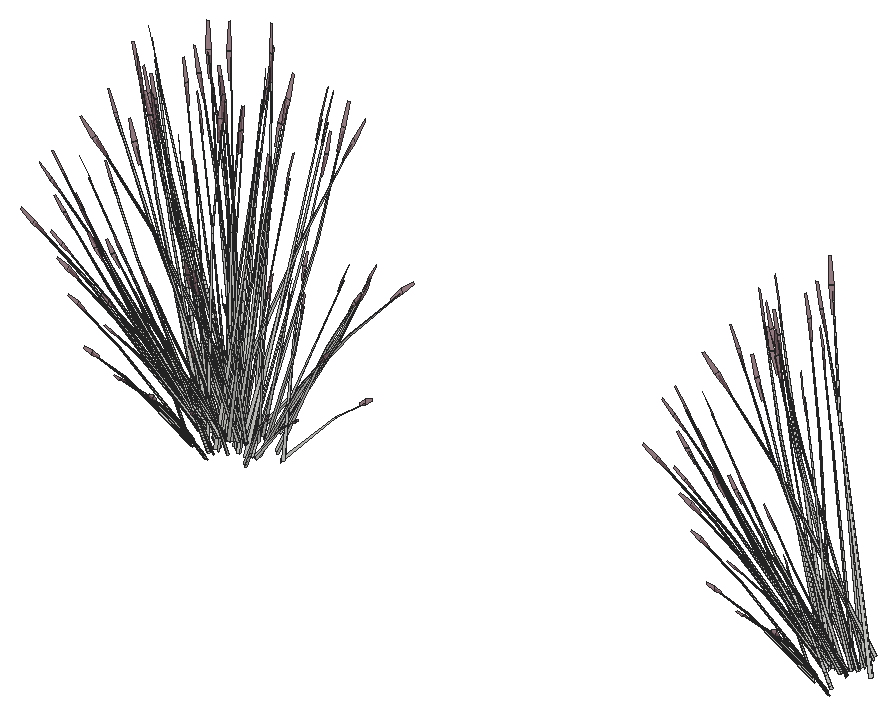
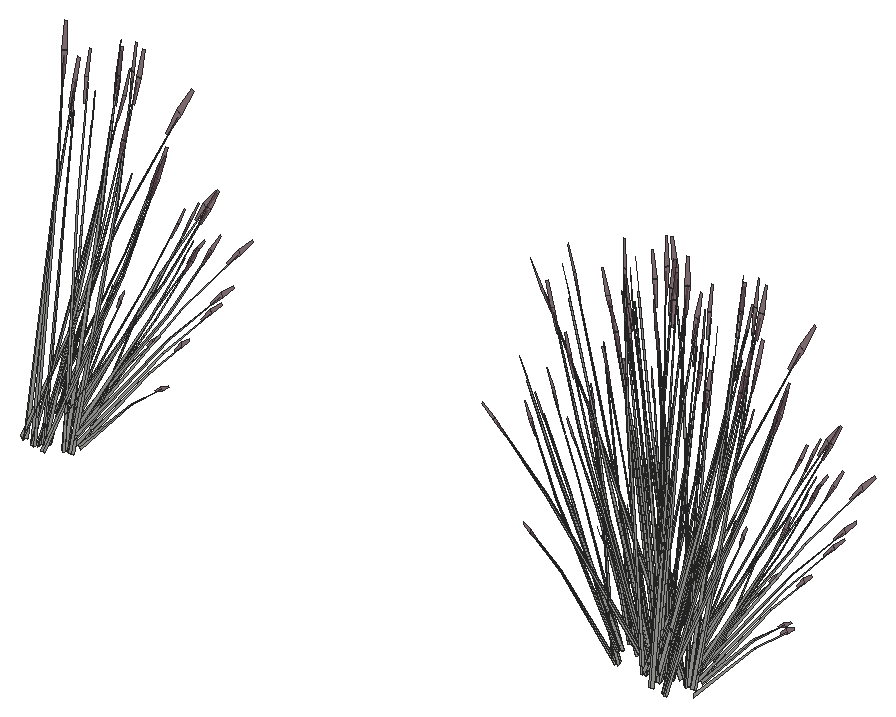
# SketchUp Ruby script. Lengths in millimetres.
U = 1.mm
M = Sketchup.active_model
def pt(a) = Geom::Point3d.new(a.map { |v| v * U })
def face(e, loops, mat)
  f = e.add_face(loops[0].map { |a| pt(a) })
  loops[1..].each { |l| e.add_face(l.map { |a| pt(a) }).erase! }
  f.material = f.back_material = mat if mat
  f
end
# faces: each face lists its corners as indices into pts; further lists are holes
def faces(e, pts, list, mat = nil) = list.each { |f| face(e, (f[0].is_a?(Array) ? f : [f]).map { |l| l.map { |i| pts[i] } }, mat) }
# xy, xz, yz: faces in a plane at the given z, y or x. An outline is a flat list of corners, or four numbers for a rectangle; further outlines are holes
def ring(l) = l.size == 4 ? [[l[0], l[1]], [l[2], l[1]], [l[2], l[3]], [l[0], l[3]]] : l.each_slice(2).to_a
def flat(e, list, mat, &to3) = list.each { |f| face(e, (f[0].is_a?(Array) ? f : [f]).map { |l| ring(l).map { |u, v| to3.(u, v) } }, mat) }
def xy(e, z, list, mat = nil) = flat(e, list, mat) { |x, y| [x, y, z] }
def xz(e, y, list, mat = nil) = flat(e, list, mat) { |x, z| [x, y, z] }
def yz(e, x, list, mat = nil) = flat(e, list, mat) { |y, z| [x, y, z] }
def lines(e, pts, list) = list.each { |a, b| e.add_line(pt(pts[a]), pt(pts[b])) }
# prism: a flat outline (further loops are holes) pulled along v
def prism(e, loops, v, mat = nil)
  f = face(e, loops, mat); d = Geom::Vector3d.new(v.map { |x| x * U })
  f.pushpull(f.normal.samedirection?(d) ? d.length : -d.length)
end
def box(e, o, s, mat = nil) = prism(e, [[o, [o[0] + s[0], o[1], o[2]], [o[0] + s[0], o[1] + s[1], o[2]], [o[0], o[1] + s[1], o[2]]]], [0, 0, s[2]], mat)
def at(x, y, z, deg = 0) = Geom::Transformation.translation(pt([x, y, z])) * Geom::Transformation.rotation(ORIGIN, Z_AXIS, deg.degrees)
def axes(o, x, y, z) = Geom::Transformation.new([*x, 0, *y, 0, *z, 0, *pt(o).to_a, 1])
def part(name) = M.definitions.add(name)
# library, detail: a bought-in or finely detailed component or shape, given as its bounding box
def library(name, o, s) = part(name).tap { |d| box(d.entities, o, s) }
def detail(e, o, s) = box(e.add_group.entities, o, s)
def put(e, d, t, mat = nil) = e.add_instance(d, t).tap { |i| i.material = mat if mat }
def group(e, t, mat = nil) = e.add_group.tap { |g| g.transformation = t; g.material = mat if mat }.entities
root = M.entities
M.materials.add("LightPink_Translucent").color = [144, 107, 117]
M.materials["LightPink_Translucent"].alpha = 0.8
c1 = part("blade")
p = [[54.7,5.3,558.8],[0,4.4,0],[2.3,11.5,0],[55.5,7.8,558.8],[58.2,7.8,558.8],[9.8,11.5,0],
  [62.9,5.7,838.2],[63,6,838.2],[63.4,6,838.2]]
faces(c1.entities,p,[[0,1,2,3],[4,5,2,3],[6,0,3,7],[7,3,4,8]])
c2 = part("seeds")
p = [[7.6,-2.7,35.1],[-0.2,-0.6,40.4],[-0.2,-0.8,0.9],[3.5,-1.8,-1.7],[7.5,-0.8,76.3],[3.7,0.2,78.9]]
faces(c2.entities,p,[[0,1,2,3],[1,0,4,5]],"LightPink_Translucent")
c3 = part("blade with seeds")
put(c3.entities,c1,at(0,0,0))
put(c3.entities,c2,axes([60.9,6.5,787.2],[1.5799,-0.05474,1.17369],[-0.12525,1.92788,0.29478],[-0.07173,-0.02425,1.56792]))
put(root,c3,axes([7452.9,4162.9,98.5],[0.28013,0.33252,1.71376],[-1.29445,0.27994,0.13857],[-0.29256,-0.52202,0.73262]))
put(root,c3,axes([7580.8,4150.6,65.8],[-0.34835,0.20963,1.43002],[-1.04325,-0.36691,-0.30754],[0.19338,-0.4563,0.61141]))
put(root,c3,axes([7540.5,4169.2,126.5],[-0.5849,-0.8421,-0.71045],[1.20401,-0.4693,0.08574],[-0.13677,-0.40688,1.00501]))
put(root,c3,axes([7443.8,4140.6,65.8],[-0.07421,0.33879,1.43002],[-1.08488,0.28361,-0.30754],[-0.25359,-0.4379,0.61141]))
put(root,c3,axes([7514.8,4121.7,37.9],[-0.20555,0.03731,1.76342],[-1.13672,-0.42002,-0.26939],[0.01907,-0.35034,0.30037]))
put(root,c3,axes([7602.3,4190.1,126.5],[0.03189,-0.95798,-0.71045],[1.34277,0.06434,0.08574],[0.14171,-0.40585,1.00501]))
put(root,c3,axes([7543.3,4151,115],[0.36946,-0.79643,-0.35414],[1.07787,0.23229,0.4572],[-0.09883,-0.32066,0.87481]))
put(root,c3,axes([7564,4177.7,98.5],[-0.22818,0.35597,1.71376],[-0.95725,-0.73667,0.13857],[0.43183,-0.45914,0.73262]))
put(root,c3,axes([10072.9,4206.3,98.5],[0.28013,0.33252,1.71376],[-1.29445,0.27994,0.13857],[-0.29256,-0.52202,0.73262]))
put(root,c3,axes([7529.3,4164.9,118.9],[-1.20468,-0.25962,-0.51099],[0.41292,-0.89013,-0.3958],[-0.11046,-0.35838,0.97773]))
put(root,c3,axes([7548.2,4108.3,70.2],[0.15721,0.60392,1.1486],[-0.87211,-0.33448,0.84392],[0.09385,-0.30923,0.25299]))
put(root,c3,axes([7595.4,4182,118.9],[-0.87728,-0.69587,-0.51099],[0.92674,-0.60943,-0.3958],[0.13348,-0.35356,0.97773]))
put(root,c3,axes([10160.5,4212.6,126.5],[-0.5849,-0.8421,-0.71045],[1.20401,-0.4693,0.08574],[-0.13677,-0.40688,1.00501]))
put(root,c3,axes([10063.8,4184,65.8],[-0.07421,0.33879,1.43002],[-1.08488,0.28361,-0.30754],[-0.25359,-0.4379,0.61141]))
put(root,c3,axes([10134.8,4165.2,37.9],[-0.20555,0.03731,1.76342],[-1.13672,-0.42002,-0.26939],[0.01907,-0.35034,0.30037]))
put(root,c3,axes([7616.4,4175.4,115],[0.82919,-0.54528,-0.35414],[0.78493,0.62262,0.4572],[0.11943,-0.31634,0.87481]))
put(root,c3,axes([7434.4,4126.7,70.2],[0.63926,0.36046,1.1486],[-0.93099,0.21668,0.84392],[-0.1992,-0.27702,0.25299]))
put(root,c3,axes([7473.5,4175.2,126.5],[-1.04497,-0.50058,-0.71045],[0.74264,-0.8772,0.08574],[-0.3786,-0.29889,1.00501]))
put(root,c3,axes([7464.4,4158.4,115],[-0.18927,-0.83419,-0.35414],[1.08199,-0.22027,0.4572],[-0.29062,-0.23905,0.87481]))
put(root,c3,axes([10163.3,4194.4,115],[0.36946,-0.79643,-0.35414],[1.07787,0.23229,0.4572],[-0.09883,-0.32066,0.87481]))
put(root,c3,axes([10149.3,4208.3,118.9],[-1.20468,-0.25962,-0.51099],[0.41292,-0.89013,-0.3958],[-0.11046,-0.35838,0.97773]))
put(root,c3,axes([7421.5,4154.3,37.9],[-0.11871,0.13643,1.76342],[-1.19964,0.29415,-0.26939],[-0.2898,-0.26759,0.30037]))
put(root,c3,axes([7471.8,4249.5,53.3],[-0.50328,-1.06202,-0.69835],[1.44974,-0.38248,-0.18329],[-0.05563,-0.35963,1.54149]))
put(root,c3,axes([7405.2,4189.2,98.5],[0.45521,0.17844,1.71376],[-0.94204,0.74856,0.13857],[-0.58713,-0.33769,0.73262]))
put(root,c3,axes([7642.7,4167.1,37.9],[-0.18342,-0.08159,1.76342],[-0.47115,-0.9115,-0.26939],[0.31784,-0.24736,0.30037]))
put(root,c3,axes([10054.4,4170.1,70.2],[0.63926,0.36046,1.1486],[-0.93099,0.21668,0.84392],[-0.1992,-0.27702,0.25299]))
put(root,c3,axes([7461.1,4175.9,118.9],[-1.20928,0.24619,-0.51099],[-0.21154,-0.93233,-0.3958],[-0.32481,-0.26718,0.97773]))
put(root,c3,axes([10093.5,4218.7,126.5],[-1.04497,-0.50058,-0.71045],[0.74264,-0.8772,0.08574],[-0.3786,-0.29889,1.00501]))
put(root,c3,axes([10084.3,4201.9,115],[-0.18927,-0.83419,-0.35414],[1.08199,-0.22027,0.4572],[-0.29062,-0.23905,0.87481]))
put(root,c3,axes([7642.5,4232.4,126.5],[0.64013,-0.81717,-0.71045],[1.12174,0.58074,0.08574],[0.38221,-0.29607,1.00501]))
put(root,c3,axes([7466.7,4171.9,60.3],[-0.7662,-1.03778,0],[1.28187,-0.57875,-0.51607],[0.29196,-0.13181,1.63711]))
put(root,c3,axes([7641.7,4222.7,118.9],[-0.31482,-0.94565,-0.51099],[1.19224,-0.16542,-0.3958],[0.34166,-0.254,0.97773]))
put(root,c3,axes([7509.5,4140.2,54.1],[-0.84686,0.59414,-0.03893],[-0.77596,-0.65071,-0.17649],[-0.05463,-0.18438,0.58215]))
put(root,c3,axes([10041.5,4197.7,37.9],[-0.11871,0.13643,1.76342],[-1.19964,0.29415,-0.26939],[-0.2898,-0.26759,0.30037]))
put(root,c3,axes([10091.8,4293,53.3],[-0.50328,-1.06202,-0.69835],[1.44974,-0.38248,-0.18329],[-0.05563,-0.35963,1.54149]))
put(root,c3,axes([10025.2,4232.7,98.5],[0.45521,0.17844,1.71376],[-0.94204,0.74856,0.13857],[-0.58713,-0.33769,0.73262]))
put(root,c3,axes([7537.1,4319.1,84.5],[1.05902,0.41762,1.51261],[-1.03748,0.89969,0.59816],[-0.46471,-0.53324,1.26806]))
put(root,c3,axes([7396.4,4245.7,51.2],[0,-1.03566,-0.49651],[1.37109,0,0],[0,-0.23588,1.57504]))
put(root,c3,axes([7493.2,4167.9,51.2],[1.14694,-0.51783,-0.49651],[0.68554,0.92854,0],[0.26122,-0.11794,1.57504]))
put(root,c3,axes([10081.1,4219.3,118.9],[-1.20928,0.24619,-0.51099],[-0.21154,-0.93233,-0.3958],[-0.32481,-0.26718,0.97773]))
put(root,c3,axes([7666.1,4213.3,65.8],[-0.4378,-0.03068,1.43002],[-0.44851,-0.8229,-0.30754],[0.53783,-0.23279,0.61141]))
put(root,c3,axes([7527.7,4221.8,52.3],[0.82544,-0.77843,-0.62353],[1.0254,0.70586,-0.16365],[0.33076,-0.19418,1.37633]))
put(root,c3,axes([7678.9,4174.9,70.2],[-0.40819,0.5272,1.1486],[-0.35086,-0.70831,0.84392],[0.33713,-0.17749,0.25299]))
put(root,c3,axes([10129.5,4183.6,54.1],[-0.84686,0.59414,-0.03893],[-0.77596,-0.65071,-0.17649],[-0.05463,-0.18438,0.58215]))
put(root,c3,axes([7664.1,4225.2,115],[1.06674,-0.14801,-0.35414],[0.28168,0.84611,0.4572],[0.30569,-0.22726,0.87481]))
put(root,c3,axes([7491.2,4256.5,56.2],[0.59459,-0.93321,-0.44739],[1.23546,0.44912,0.21531],[0,-0.21512,1.43643]))
put(root,c3,axes([7400.7,4195.7,115],[-0.69728,-0.64842,-0.35414],[0.79619,-0.61382,0.4572],[-0.40453,-0.09339,0.87481]))
put(root,c3,axes([7505,4244.7,67.7],[-0.1428,-1.18174,-0.29095],[1.48733,-0.07145,-0.50002],[0.26191,-0.15741,1.59708]))
put(root,c3,axes([7411.4,4246.3,51.5],[0.85545,-0.64616,-0.30978],[0.85545,0.64616,0.30978],[0,-0.20813,1.38974]))
put(root,c3,axes([7402.6,4167.6,54.1],[-0.35352,0.84566,-0.03893],[-1.08806,-0.26014,-0.17649],[-0.1652,-0.13832,0.58215]))
put(root,c3,axes([7487.4,4276.2,67.7],[-1.38012,-0.49416,-0.29095],[0.66454,-1.04299,-0.50002],[-0.04337,-0.25608,1.59708]))
put(root,c3,axes([10157.1,4362.5,84.5],[1.05902,0.41762,1.51261],[-1.03748,0.89969,0.59816],[-0.46471,-0.53324,1.26806]))
put(root,c3,axes([7387.7,4265.7,60.3],[-1.53239,0,0],[0,-1.1575,-0.51607],[0,-0.26363,1.63711]))
put(root,c3,axes([7394.3,4213.2,65.8],[0.23927,0.28834,1.43002],[-0.55135,0.78376,-0.30754],[-0.56612,-0.18733,0.61141]))
put(root,c3,axes([10016.4,4289.2,51.2],[0,-1.03566,-0.49651],[1.37109,0,0],[0,-0.23588,1.57504]))
put(root,c3,axes([7500,4178.3,51.5],[1.14332,0.25625,-0.30978],[-0.28787,0.90242,0.30978],[0.23049,-0.10406,1.38974]))
put(root,c3,axes([7419.4,4206.7,126.5],[-1.22504,-0.02494,-0.71045],[0.08228,-1.05005,0.08574],[-0.51899,-0.11081,1.00501]))
put(root,c3,axes([10020.7,4239.1,115],[-0.69728,-0.64842,-0.35414],[0.79619,-0.61382,0.4572],[-0.40453,-0.09339,0.87481]))
put(root,c3,axes([7417.9,4257.9,59.2],[-1.1399,0.87071,0.30756],[-1.1406,-0.86155,-0.36492],[-0.03981,-0.24727,1.64885]))
put(root,c3,axes([10031.3,4289.8,51.5],[0.85545,-0.64616,-0.30978],[0.85545,0.64616,0.30978],[0,-0.20813,1.38974]))
put(root,c3,axes([10022.6,4211.1,54.1],[-0.35352,0.84566,-0.03893],[-1.08806,-0.26014,-0.17649],[-0.1652,-0.13832,0.58215]))
put(root,c3,axes([10107.4,4319.6,67.7],[-1.38012,-0.49416,-0.29095],[0.66454,-1.04299,-0.50002],[-0.04337,-0.25608,1.59708]))
put(root,c3,axes([7509.9,4268.3,61.8],[1.3808,0.50196,0.24065],[-0.66454,1.04299,0.50002],[0,-0.24043,1.60543]))
put(root,c3,axes([10007.7,4309.1,60.3],[-1.53239,0,0],[0,-1.1575,-0.51607],[0,-0.26363,1.63711]))
put(root,c3,axes([7496.3,4304.1,61.9],[0.32481,-1.2272,-0.23429],[1.54007,0.21392,0.51271],[-0.26911,-0.16947,1.5644]))
put(root,c3,axes([10014.3,4256.6,65.8],[0.23927,0.28834,1.43002],[-0.55135,0.78376,-0.30754],[-0.56612,-0.18733,0.61141]))
put(root,c3,axes([7409.1,4212.1,118.9],[-0.88986,0.68603,-0.51099],[-0.77932,-0.72471,-0.3958],[-0.45212,-0.10438,0.97773]))
put(root,c3,axes([7358.2,4235.1,70.2],[0.78239,-0.07411,1.1486],[-0.49629,0.65296,0.84392],[-0.38663,-0.09795,0.25299]))
put(root,c3,axes([10039.4,4250.1,126.5],[-1.22504,-0.02494,-0.71045],[0.08228,-1.05005,0.08574],[-0.51899,-0.11081,1.00501]))
put(root,c3,axes([7498.6,4250.5,69],[-1.33077,0.06393,0.44739],[-0.12035,-1.06125,-0.21531],[0.23824,-0.10756,1.43643]))
put(root,c3,axes([7411.3,4270.2,63],[0,1.03566,0.49651],[-1.37109,0,0],[0,-0.23588,1.57504]))
put(root,c3,axes([7655.8,4276,118.9],[0.332,-0.94205,-0.51099],[1.13828,0.3229,-0.3958],[0.45829,-0.08638,0.97773]))
put(root,c3,axes([7610.1,4178.6,60.4],[0.7662,-1.03778,0],[1.28187,0.57875,-0.51607],[0.29196,0.13181,1.63711]))
put(root,c3,axes([7380.8,4230.7,98.5],[0.50831,-0.02346,1.71376],[-0.33721,1.01661,0.13857],[-0.72439,-0.06288,0.73262]))
put(root,c3,axes([7493.6,4291.4,56.2],[-0.73619,-0.86927,-0.44739],[1.11511,-0.61213,0.21531],[-0.23824,-0.10756,1.43643]))
put(root,c3,axes([7497.4,4260.2,60],[0.53281,1.15808,0.45755],[-1.52239,0.4027,0.17955],[0.01861,-0.2128,1.58856]))
put(root,c3,axes([7686.7,4282.8,50.4],[-0.7893,0.12429,1.41583],[-0.12563,-0.9893,0.08104],[0.55282,-0.14974,0.80566]))
put(root,c3,axes([7723.2,4260.5,57.4],[-0.75977,-0.66224,-0.06488],[0.83212,-0.6068,-0.29416],[0.23578,-0.04272,0.97024]))
put(root,c3,axes([10037.9,4301.4,59.2],[-1.1399,0.87071,0.30756],[-1.1406,-0.86155,-0.36492],[-0.03981,-0.24727,1.64885]))
put(root,c3,axes([7490.6,4283.4,69],[-0.59459,0.93321,0.44739],[-1.23546,-0.44912,-0.21531],[0,-0.21512,1.43643]))
put(root,c3,axes([7546.1,4262.7,56],[0,-1.19833,0],[1.53239,0,0],[0,0,1.79456]))
put(root,c3,axes([7593.3,4192.4,63],[-1.14694,-0.51783,0.49651],[0.68554,-0.92854,0],[0.26122,0.11794,1.57504]))
put(root,c3,axes([7650.3,4284.7,126.5],[1.07686,-0.45739,-0.71045],[0.60013,0.94154,0.08574],[0.52031,-0.10696,1.00501]))
put(root,c3,axes([10116.3,4347.5,61.9],[0.32481,-1.2272,-0.23429],[1.54007,0.21392,0.51271],[-0.26911,-0.16947,1.5644]))
put(root,c3,axes([10029.1,4255.5,118.9],[-0.88986,0.68603,-0.51099],[-0.77932,-0.72471,-0.3958],[-0.45212,-0.10438,0.97773]))
put(root,c3,axes([7476.8,4299.8,52.3],[-1.27479,-0.1698,-0.62353],[0.26901,-1.04736,-0.16365],[-0.38043,-0.12691,1.37633]))
put(root,c3,axes([7527.7,4243.5,60],[-1.01611,0.93987,0.45755],[-1.20717,-0.82966,0.17955],[0.24496,-0.0938,1.58856]))
put(root,c3,axes([9978.2,4278.6,70.2],[0.78239,-0.07411,1.1486],[-0.49629,0.65296,0.84392],[-0.38663,-0.09795,0.25299]))
put(root,c3,axes([7555.8,4286.3,58.4],[-1.1399,-0.8914,-0.06131],[1.1406,-0.89194,0],[-0.03981,-0.03113,1.75571]))
put(root,c3,axes([7482.9,4204.2,62.8],[-0.35402,1.02926,0.17642],[-1.29548,-0.29127,0.35086],[0.22379,-0.00501,1.60407]))
put(root,c3,axes([10031.3,4313.6,63],[0,1.03566,0.49651],[-1.37109,0,0],[0,-0.23588,1.57504]))
put(root,c3,axes([7469.2,4225.3,40.5],[-1.20625,0.41464,1.28929],[-0.38394,-1.1897,0.50096],[0.74071,0.01979,1.46642]))
put(root,c3,axes([7551.6,4233.3,66.5],[0.23642,-0.92427,0.1448],[1.15506,0.16044,-0.41347],[0.21021,0.09491,1.26744]))
put(root,c3,axes([7500.8,4289,60],[1.54892,0.2182,0.45755],[-0.31522,1.23236,0.17955],[-0.22636,-0.119,1.58856]))
put(root,c3,axes([7708.5,4266.3,37.9],[-0.06405,-0.15723,1.76342],[0.44421,-0.91974,-0.26939],[0.4481,-0.01323,0.30037]))
put(root,c3,axes([10000.8,4274.1,98.5],[0.50831,-0.02346,1.71376],[-0.33721,1.01661,0.13857],[-0.72439,-0.06288,0.73262]))
put(root,c3,axes([10113.6,4334.8,56.2],[-0.73619,-0.86927,-0.44739],[1.11511,-0.61213,0.21531],[-0.23824,-0.10756,1.43643]))
put(root,c3,axes([7372.7,4262.3,37.9],[0.03108,0.16322,1.76342],[-0.62654,0.85237,-0.26939],[-0.44504,-0.04296,0.30037]))
put(root,c3,axes([7539,4239.4,69],[-0.73619,-0.86927,0.44739],[1.11511,-0.61213,-0.21531],[0.23824,0.10756,1.43643]))
put(root,c3,axes([7442.4,4340.4,51.5],[-0.28787,-0.90242,-0.30978],[1.14332,-0.25625,0.30978],[-0.23049,-0.10406,1.38974]))
put(root,c3,axes([10110.6,4326.8,69],[-0.59459,0.93321,0.44739],[-1.23546,-0.44912,-0.21531],[0,-0.21512,1.43643]))
put(root,c3,axes([7479.7,4339,62.8],[1.31687,-0.27488,0.17642],[0.32517,1.02297,0.35086],[-0.11745,-0.14905,1.60407]))
put(root,c3,axes([7548.6,4240.9,67.7],[1.23732,-0.68758,-0.29095],[0.8228,0.97154,-0.50002],[0.30528,0.09867,1.59708]))
put(root,c3,axes([7673.5,4286.9,115],[1.01846,0.28891,-0.35414],[-0.29705,0.84289,0.4572],[0.41005,-0.07729,0.87481]))
put(root,c3,axes([7434.3,4350.2,51.2],[-1.14694,-0.51783,-0.49651],[0.68554,-0.92854,0],[-0.26122,-0.11794,1.57504]))
put(root,c3,axes([7627.8,4194.5,51.2],[1.14694,0.51783,-0.49651],[-0.68554,0.92854,0],[0.26122,0.11794,1.57504]))
put(root,c3,axes([10096.8,4343.3,52.3],[-1.27479,-0.1698,-0.62353],[0.26901,-1.04736,-0.16365],[-0.38043,-0.12691,1.37633]))
put(root,c3,axes([7369.5,4252.8,115],[-1.01846,-0.28891,-0.35414],[0.29705,-0.84289,0.4572],[-0.41005,0.07729,0.87481]))
put(root,c3,axes([7572.5,4269.5,56],[1.37109,0,0],[0,1.07219,0],[0,0,1.78407]))
put(root,c3,axes([10175.8,4329.7,58.4],[-1.1399,-0.8914,-0.06131],[1.1406,-0.89194,0],[-0.03981,-0.03113,1.75571]))
put(root,c3,axes([7513.5,4303.8,67.7],[-1.23732,0.68758,-0.29095],[-0.8228,-0.97154,-0.50002],[-0.30528,-0.09867,1.59708]))
put(root,c3,axes([7582.4,4205.6,62.8],[-1.31687,0.27488,0.17642],[-0.32517,-1.02297,0.35086],[0.11745,0.14905,1.60407]))
put(root,c3,axes([7603,4260.4,98.5],[-0.50831,0.02346,1.71376],[0.33721,-1.01661,0.13857],[0.72439,0.06288,0.73262]))
put(root,c3,axes([7619.7,4204.3,51.5],[0.28787,0.90242,-0.30978],[-1.14332,0.25625,0.30978],[0.23049,0.10406,1.38974]))
put(root,c3,axes([10120.8,4332.5,60],[1.54892,0.2182,0.45755],[-0.31522,1.23236,0.17955],[-0.22636,-0.119,1.58856]))
